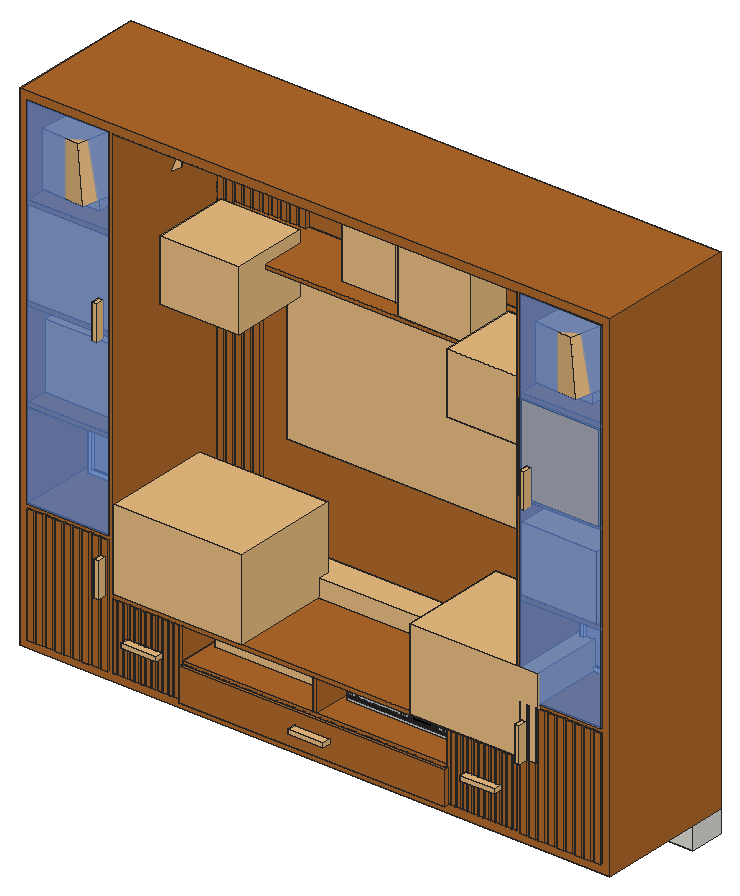
# SketchUp Ruby script. Lengths in millimetres.
U = 1.mm
M = Sketchup.active_model
def pt(a) = Geom::Point3d.new(a.map { |v| v * U })
def face(e, loops, mat)
  f = e.add_face(loops[0].map { |a| pt(a) })
  loops[1..].each { |l| e.add_face(l.map { |a| pt(a) }).erase! }
  f.material = f.back_material = mat if mat
  f
end
# faces: each face lists its corners as indices into pts; further lists are holes
def faces(e, pts, list, mat = nil) = list.each { |f| face(e, (f[0].is_a?(Array) ? f : [f]).map { |l| l.map { |i| pts[i] } }, mat) }
# xy, xz, yz: faces in a plane at the given z, y or x. An outline is a flat list of corners, or four numbers for a rectangle; further outlines are holes
def ring(l) = l.size == 4 ? [[l[0], l[1]], [l[2], l[1]], [l[2], l[3]], [l[0], l[3]]] : l.each_slice(2).to_a
def flat(e, list, mat, &to3) = list.each { |f| face(e, (f[0].is_a?(Array) ? f : [f]).map { |l| ring(l).map { |u, v| to3.(u, v) } }, mat) }
def xy(e, z, list, mat = nil) = flat(e, list, mat) { |x, y| [x, y, z] }
def xz(e, y, list, mat = nil) = flat(e, list, mat) { |x, z| [x, y, z] }
def yz(e, x, list, mat = nil) = flat(e, list, mat) { |y, z| [x, y, z] }
def lines(e, pts, list) = list.each { |a, b| e.add_line(pt(pts[a]), pt(pts[b])) }
# prism: a flat outline (further loops are holes) pulled along v
def prism(e, loops, v, mat = nil)
  f = face(e, loops, mat); d = Geom::Vector3d.new(v.map { |x| x * U })
  f.pushpull(f.normal.samedirection?(d) ? d.length : -d.length)
end
def box(e, o, s, mat = nil) = prism(e, [[o, [o[0] + s[0], o[1], o[2]], [o[0] + s[0], o[1] + s[1], o[2]], [o[0], o[1] + s[1], o[2]]]], [0, 0, s[2]], mat)
def at(x, y, z, deg = 0) = Geom::Transformation.translation(pt([x, y, z])) * Geom::Transformation.rotation(ORIGIN, Z_AXIS, deg.degrees)
def axes(o, x, y, z) = Geom::Transformation.new([*x, 0, *y, 0, *z, 0, *pt(o).to_a, 1])
def part(name) = M.definitions.add(name)
# library, detail: a bought-in or finely detailed component or shape, given as its bounding box
def library(name, o, s) = part(name).tap { |d| box(d.entities, o, s) }
def detail(e, o, s) = box(e.add_group.entities, o, s)
def put(e, d, t, mat = nil) = e.add_instance(d, t).tap { |i| i.material = mat if mat }
def group(e, t, mat = nil) = e.add_group.tap { |g| g.transformation = t; g.material = mat if mat }.entities
root = M.entities
M.materials.add("Material__1").color = [190, 136, 85]
M.materials.add("Material__2").color = [51, 42, 44]
M.materials.add("Material__3").color = [119, 136, 107]
M.materials.add("Paintiing ").color = [206, 175, 155]
M.materials.add("[0131_Silver]").color = [192, 192, 192]
M.materials.add("[0136_Charcoal]").color = [35, 35, 35]
M.materials.add("[0137_Black]").color = [0, 0, 0]
M.materials.add("[Marble Carrara Gold Floor Tile]").color = [225, 223, 217]
M.materials.add("[Translucent Glass Blue]").color = [100, 149, 237]
M.materials["[Translucent Glass Blue]"].alpha = 0.5
M.materials.add("[Wood Bamboo]").color = [177, 105, 43]
c1 = part("Circular disc")
prism(c1.entities,[[[0,76.2,-25],[2.6,95.9,-25],[10.2,114.3,-25],[22.3,130.1,-25],[38.1,142.2,-25],[56.5,149.8,-25],[76.2,152.4,-25],[95.9,149.8,-25],[114.3,142.2,-25],[130.1,130.1,-25],[142.2,114.3,-25],[149.8,95.9,-25],[152.4,76.2,-25],[149.8,56.5,-25],[142.2,38.1,-25],[130.1,22.3,-25],[114.3,10.2,-25],[95.9,2.6,-25],[76.2,0,-25],[56.5,2.6,-25],[38.1,10.2,-25],[22.3,22.3,-25],[10.2,38.1,-25],[2.6,56.5,-25]]],[0,0,13])
c2 = library("1-POIGNEE CLC2\#1",[-77,-9.5,0],[154,19,36])
c3 = library("1-POIGNEE CLC2\#2",[-77,-9.5,0],[154,19,36])
c4 = library("1-POIGNEE CLC2\#3",[-77,-9.5,0],[154,19,36])
c5 = library("download?mid=50c7180b9fccec56d493bfe20f94b6ab&ctyp=sp&cv=p8.",[3795.5,1113.3,453.6],[1898.6,14.5,1067.8])
c6 = library("cay+chuoi",[682.9,499.4,13.3],[1066,1159.4,897.8])
c7 = library("\#2",[-3043.7,-3043.7,2890.5],[6087.4,6087.4,441.9])
c8 = library("\#4",[-4912.8,-5236.5,-6012.5],[10484.7,6383.2,12002.4])
c9 = part("\#3")
put(c9.entities,c8,axes([-9.5,7866.8,0],[1.36765,0,0],[0,1.36765,0],[0,0,1.36765]),"Material__3")
c10 = library("\#1",[-4421.5,-4421.5,0],[8843,8843,3556])
c11 = part("9")
put(c11.entities,c7,at(-506.5,-626.4,0),"Material__2")
put(c11.entities,c9,axes([448.8,-828,1023.3],[0.29694,0.9549,0],[-0.21403,0.06656,0.97456],[0.9306,-0.28939,0.22414]))
put(c11.entities,c10,at(-506.5,-626.4,0),"Material__1")
c12 = library("Hanging potted plant",[2125.6,-54.2,204.6],[849,690.2,1168.3])
c13 = library("Plant (3)",[-393.8,66.9,0],[2990,2448.2,4692.7])
c14 = library("Pot Wired",[-4344.5,-4889.6,-19],[9129.4,9129.4,7192.3])
c15 = library("Seated statue",[0,0,0],[467.3,421.3,661.2])
c16 = part("Framed panel")
xy(c16.entities,0,[[[0,0,1153.7,1374.2],[66.8,66.8,1086.8,1307.4]]])
xy(c16.entities,0,[[66.8,66.8,1086.8,1307.4]],"Paintiing ")
xy(c16.entities,10,[[[0,0,1153.7,1374.2],[66.8,66.8,1086.8,1307.4]]])
xz(c16.entities,0,[[0,0,1153.7,10]])
xz(c16.entities,66.8,[[66.8,0,1086.8,10]])
xz(c16.entities,1307.4,[[66.8,0,1086.8,10]])
xz(c16.entities,1374.2,[[0,0,1153.7,10]])
yz(c16.entities,0,[[0,0,1374.2,10]])
yz(c16.entities,66.8,[[66.8,0,1307.4,10]])
yz(c16.entities,1086.8,[[66.8,0,1307.4,10]])
yz(c16.entities,1153.7,[[0,0,1374.2,10]])
c17 = library("SetUp-Box",[-7.9,-1.3,-4],[171.7,230.9,39.1])
c18 = library("Ganesha+-+An+Do+Giao",[214.1,-280.3,-3.5],[241.1,146.8,312])
c19 = library("Samsung+soundbar",[-449.8,4.4,0],[1488,131,78.2])
c20 = part("Untitled")
xy(c20.entities,695.4,[[-2447.8,-1052.2,-473,-61.6]],"[0131_Silver]")
xy(c20.entities,720.8,[[-2447.8,-1058.5,-473,-1052.2]],"[0136_Charcoal]")
xy(c20.entities,740.9,[[-1374.3,-1058.5,-1037.8,-1052.2]],"[0136_Charcoal]")
xy(c20.entities,758.1,[[-913.8,-1077.6,-831.3,-1058.5]],"[0131_Silver]")
xy(c20.entities,758.3,[[-636.9,-1077.6,-579.8,-1058.5]],"[0131_Silver]")
xy(c20.entities,762.4,[[-1518.7,-1077.6,-1436.1,-1058.5]],"[0131_Silver]")
xy(c20.entities,762.6,[[-714.1,-1077.6,-663.3,-1058.5]],"[0131_Silver]")
xy(c20.entities,762.9,[[-2398.3,-1077.6,-2315.7,-1058.5]],"[0131_Silver]")
xy(c20.entities,765.2,[[-807.4,-1077.6,-743.9,-1058.5]],"[0131_Silver]")
xy(c20.entities,768.4,[[-707.6,-1077.6,-669.5,-1064.9]],"[0131_Silver]")
xy(c20.entities,774.7,[[-707.6,-1077.6,-669.5,-1064.9]],"[0131_Silver]")
xy(c20.entities,781.5,[[-1518.7,-1077.6,-1436.1,-1058.5]],"[0131_Silver]")
xy(c20.entities,781.6,[[-714.1,-1077.6,-663.3,-1058.5]],"[0131_Silver]")
xy(c20.entities,781.9,[[-2398.3,-1077.6,-2315.7,-1058.5]],"[0131_Silver]")
xy(c20.entities,783.5,[[-913.8,-1077.6,-831.3,-1058.5]],"[0131_Silver]")
xy(c20.entities,783.7,[[-636.9,-1077.6,-634,-1058.5],[-634,-1077.6,-631.2,-1058.5],[-631.2,-1077.6,-586.7,-1058.5],[-586.7,-1077.6,-583.2,-1058.5],[-583.2,-1077.6,-579.8,-1058.5]],"[0131_Silver]")
xy(c20.entities,784.3,[[-807.4,-1077.6,-743.9,-1058.5]],"[0131_Silver]")
xy(c20.entities,791.7,[[-1374.3,-1058.5,-1037.8,-1052.2]],"[0136_Charcoal]")
xy(c20.entities,835.2,[[-2425.6,-1058.5,-488.8,-1052.2]],"[0136_Charcoal]")
xy(c20.entities,853.4,[[-2426.6,-1052.2,-502.6,-61.6]],"[0131_Silver]")
xz(c20.entities,-1077.6,[[-913.8,758.1,-831.3,783.5],[-636.9,758.3,-636.9,783.7,-634,783.7,-634,764.7,-583.2,764.7,-583.2,783.7,-579.8,783.7,-579.8,758.3],[-1518.7,762.4,-1436.1,781.5],[[-714.1,762.6,-663.3,781.6],[-707.6,768.4,-669.5,774.7]],[-2398.3,762.9,-2315.7,781.9],
  [-807.4,765.2,-743.9,784.3],[-631.2,777.4,-586.7,783.7]],"[0131_Silver]")
xz(c20.entities,-1058.5,[[-2259.9,752,-1548.7,790.1]],"[0131_Silver]")
xz(c20.entities,-1058.5,[[[-2447.8,720.8,-2447.8,816,-2447.6,818.8,-2447,821.5,-2446,824.1,-2444.7,826.5,-2443,828.7,-2441.1,830.7,-2438.9,832.4,-2436.4,833.7,-2433.8,834.7,-2431.1,835.2,-2428.3,835.4,-2425.6,835.2,-488.8,835.2,-486.5,835.1,-484.1,834.5,-481.9,833.7,-479.9,832.5,-478,831.1,-476.4,829.4,-475,827.4,-473.9,825.3,-473.2,823.1,-472.7,820.7,-472.7,818.4,-473,816,-473,720.8],[-2259.9,752,-1548.7,790.1],[-1374.3,740.9,-1037.8,791.7],[-913.8,758.1,-831.3,783.5],[-2398.3,762.9,-2315.7,781.9],[-1518.7,762.4,-1436.1,781.5],[-636.9,758.3,-579.8,783.7],[-807.4,765.2,-743.9,784.3],[-714.1,762.6,-663.3,781.6]]],"[0136_Charcoal]")
xz(c20.entities,-1052.2,[[-2447.8,695.4,-473,720.8],[-2436.4,833.7,-2433.8,834.7,-2431.1,835.2,-2428.3,835.4,-2425.6,835.2,-488.8,835.2,-486.5,835.1,-484.1,834.5,-484.1,847.2,-485.5,848.2,-486.9,849.1,-488.3,849.9,-489.8,850.6,-491.3,851.2,-492.9,851.8,-494.5,852.3,-496.1,852.7,-497.7,853,-499.3,853.2,-500.9,853.3,-502.6,853.4,-2426.6,853.4,-2428.2,853.2,-2429.8,852.9,-2431.3,852.3,-2432.6,851.4,-2433.9,850.4,-2434.9,849.2,-2435.7,847.8,-2436.4,846.3,-2436.8,844.8,-2436.9,843.2,-2436.8,841.6,-2436.4,840]],"[0131_Silver]")
xz(c20.entities,-1052.2,[[-1374.3,740.9,-1037.8,791.7]],"[0137_Black]")
xz(c20.entities,-61.6,[[-2447.8,695.4,-2447.8,816,-2447.6,818.8,-2447,821.5,-2446,824.1,-2444.7,826.5,-2443,828.7,-2441.1,830.7,-2438.9,832.4,-2436.4,833.7,-2433.8,834.7,-2431.1,835.2,-2428.3,835.4,-2425.6,835.2,-488.8,835.2,-486.5,835.1,-484.1,834.5,-481.9,833.7,-479.9,832.5,-478,831.1,-476.4,829.4,-475,827.4,-473.9,825.3,-473.2,823.1,-472.7,820.7,-472.7,818.4,-473,816,-473,695.4],[-2436.4,833.7,-2436.4,840,-2436.8,841.6,-2436.9,843.2,-2436.8,844.8,-2436.4,846.3,-2435.7,847.8,-2434.9,849.2,-2433.9,850.4,-2432.6,851.4,-2431.3,852.3,-2429.8,852.9,-2428.2,853.2,-2426.6,853.4,-502.6,853.4,-500.9,853.3,-499.3,853.2,-497.7,853,-496.1,852.7,-494.5,852.3,-492.9,851.8,-491.3,851.2,-489.8,850.6,-488.3,849.9,-486.9,849.1,-485.5,848.2,-484.1,847.2,-484.1,834.5,-486.5,835.1,-488.8,835.2,-2425.6,835.2,-2428.3,835.4,-2431.1,835.2,-2433.8,834.7]],"[0131_Silver]")
yz(c20.entities,-2447.8,[[-1052.2,695.4,-61.6,727.1],[-1058.5,720.8,-1052.2,720.8,-1052.2,727.1,-61.6,727.1,-61.6,816,-1058.5,816]],"[0131_Silver]")
yz(c20.entities,-2436.4,[[-1052.2,833.7,-61.6,840]],"[0131_Silver]")
yz(c20.entities,-2398.3,[[-1077.6,762.9,-1058.5,781.9]],"[0131_Silver]")
yz(c20.entities,-2315.7,[[-1077.6,762.9,-1058.5,781.9]],"[0131_Silver]")
yz(c20.entities,-1518.7,[[-1077.6,762.4,-1058.5,781.5]],"[0131_Silver]")
yz(c20.entities,-1436.1,[[-1077.6,762.4,-1058.5,781.5]],"[0131_Silver]")
yz(c20.entities,-1374.3,[[-1058.5,740.9,-1052.2,791.7]],"[0136_Charcoal]")
yz(c20.entities,-1037.8,[[-1058.5,740.9,-1052.2,791.7]],"[0136_Charcoal]")
yz(c20.entities,-913.8,[[-1077.6,758.1,-1058.5,783.5]],"[0131_Silver]")
yz(c20.entities,-831.3,[[-1077.6,758.1,-1058.5,783.5]],"[0131_Silver]")
yz(c20.entities,-807.4,[[-1077.6,765.2,-1058.5,784.3]],"[0131_Silver]")
yz(c20.entities,-743.9,[[-1077.6,765.2,-1058.5,784.3]],"[0131_Silver]")
yz(c20.entities,-714.1,[[-1077.6,762.6,-1058.5,781.6]],"[0131_Silver]")
yz(c20.entities,-707.6,[[-1077.6,768.4,-1064.9,774.7]],"[0131_Silver]")
yz(c20.entities,-669.5,[[-1077.6,768.4,-1064.9,774.7]],"[0131_Silver]")
yz(c20.entities,-663.3,[[-1077.6,762.6,-1058.5,781.6]],"[0131_Silver]")
yz(c20.entities,-636.9,[[-1077.6,758.3,-1058.5,783.7]],"[0131_Silver]")
yz(c20.entities,-579.8,[[-1077.6,758.3,-1058.5,783.7]],"[0131_Silver]")
yz(c20.entities,-484.1,[[-1052.2,834.5,-61.6,847.2]],"[0131_Silver]")
yz(c20.entities,-473,[[-1052.2,695.4,-61.6,727.1],[-1058.5,720.8,-1058.5,816,-61.6,816,-61.6,727.1,-1052.2,727.1,-1052.2,720.8]],"[0131_Silver]")
yz(c20.entities,-472.7,[[-1058.5,818.4,-61.6,820.7]],"[0131_Silver]")
p = [[-2447.8,-1058.5,816],[-2447.8,-61.6,816],[-2447.6,-61.6,818.8],[-2447.6,-1058.5,818.8],[-472.7,-1058.5,818.4],[-472.7,-61.6,818.4],
  [-473,-61.6,816],[-473,-1058.5,816],[-2447,-61.6,821.5],[-2447,-1058.5,821.5],[-473.2,-1058.5,823.1],[-473.2,-61.6,823.1],
  [-472.7,-61.6,820.7],[-472.7,-1058.5,820.7],[-2446,-61.6,824.1],[-2446,-1058.5,824.1],[-473.9,-1058.5,825.3],[-473.9,-61.6,825.3],
  [-2444.7,-61.6,826.5],[-2444.7,-1058.5,826.5],[-475,-1058.5,827.4],[-475,-61.6,827.4],[-2443,-61.6,828.7],[-2443,-1058.5,828.7],
  [-476.4,-1058.5,829.4],[-476.4,-61.6,829.4],[-2441.1,-61.6,830.7],[-2441.1,-1058.5,830.7],[-478,-1058.5,831.1],[-478,-61.6,831.1],
  [-2438.9,-61.6,832.4],[-2438.9,-1058.5,832.4],[-479.9,-1058.5,832.5],[-479.9,-61.6,832.5],[-2436.4,-61.6,833.7],[-2436.4,-1052.2,833.7],
  [-2436.4,-1058.5,833.7],[-481.9,-1058.5,833.7],[-481.9,-61.6,833.7],[-2433.8,-1052.2,834.7],[-2433.8,-1058.5,834.7],[-484.1,-1052.2,834.5],
  [-484.1,-61.6,834.5],[-484.1,-1058.5,834.5],[-486.5,-1052.2,835.1],[-486.5,-1058.5,835.1],[-2431.1,-1052.2,835.2],[-2431.1,-1058.5,835.2],
  [-488.8,-1052.2,835.2],[-488.8,-1058.5,835.2],[-2428.3,-1052.2,835.4],[-2428.3,-1058.5,835.4],[-2425.6,-1052.2,835.2],[-2425.6,-1058.5,835.2],
  [-2436.8,-61.6,841.6],[-2436.4,-61.6,840],[-2436.4,-1052.2,840],[-2436.8,-1052.2,841.6],[-2436.9,-61.6,843.2],[-2436.9,-1052.2,843.2],
  [-2436.8,-61.6,844.8],[-2436.8,-1052.2,844.8],[-2436.4,-61.6,846.3],[-2436.4,-1052.2,846.3],[-2435.7,-61.6,847.8],[-2435.7,-1052.2,847.8],
  [-484.1,-61.6,847.2],[-485.5,-61.6,848.2],[-485.5,-1052.2,848.2],[-484.1,-1052.2,847.2],[-2434.9,-61.6,849.2],[-2434.9,-1052.2,849.2],
  [-486.9,-61.6,849.1],[-486.9,-1052.2,849.1],[-488.3,-61.6,849.9],[-488.3,-1052.2,849.9],[-2433.9,-61.6,850.4],[-2433.9,-1052.2,850.4],
  [-489.8,-61.6,850.6],[-489.8,-1052.2,850.6],[-2432.6,-61.6,851.4],[-2432.6,-1052.2,851.4],[-491.3,-61.6,851.2],[-491.3,-1052.2,851.2],
  [-492.9,-61.6,851.8],[-492.9,-1052.2,851.8],[-2431.3,-61.6,852.3],[-2431.3,-1052.2,852.3],[-494.5,-61.6,852.3],[-494.5,-1052.2,852.3],
  [-2429.8,-61.6,852.9],[-2429.8,-1052.2,852.9],[-496.1,-61.6,852.7],[-496.1,-1052.2,852.7],[-497.7,-61.6,853],[-497.7,-1052.2,853],
  [-2428.2,-61.6,853.2],[-2428.2,-1052.2,853.2],[-499.3,-61.6,853.2],[-499.3,-1052.2,853.2],[-2426.6,-61.6,853.4],[-2426.6,-1052.2,853.4],
  [-500.9,-61.6,853.3],[-500.9,-1052.2,853.3],[-502.6,-61.6,853.4],[-502.6,-1052.2,853.4],[-486.5,-620.4,835.1],[-488.8,-620.4,835.2],
  [-2425.6,-620.4,835.2],[-2428.3,-620.4,835.4],[-2431.1,-620.4,835.2],[-2433.8,-620.4,834.7]]
faces(c20.entities,p,[[0,1,2,3],[4,5,6,7],[3,2,8,9],[10,11,12,13],[9,8,14,15],[16,17,11,10],[15,14,18,19],[20,21,17,16],
  [19,18,22,23],[24,25,21,20],[23,22,26,27],[28,29,25,24],[27,26,30,31],[32,33,29,28],[31,30,34,35,36],[37,38,33,32],
  [41,42,38,37,43],[54,55,56,57],[58,54,57,59],[60,58,59,61],[62,60,61,63],[64,62,63,65],[66,67,68,69],[70,64,65,71],
  [67,72,73,68],[72,74,75,73],[76,70,71,77],[74,78,79,75],[80,76,77,81],[78,82,83,79],[82,84,85,83],[86,80,81,87],
  [84,88,89,85],[90,86,87,91],[88,92,93,89],[92,94,95,93],[96,90,91,97],[94,98,99,95],[100,96,97,101],[98,102,103,99],
  [102,104,105,103]],"[0131_Silver]")
faces(c20.entities,p,[[39,35,36,40],[41,44,45,43],[46,39,40,47],[44,48,49,45],[50,46,47,51],[52,50,51,53]])
lines(c20.entities,p,[[106,44],[107,48],[108,52],[109,50],[110,46],[111,39]])
c21 = library("1-POIGNEE CLC2\#4",[-77,-9.5,0],[154,19,36])
c22 = part("louvers")
box(c22.entities,[0,-2,0],[18.7,2,291])
box(c22.entities,[24.8,-2,0],[18.7,2,291])
box(c22.entities,[49.5,-2,0],[18.7,2,291])
box(c22.entities,[74.3,-2,0],[18.7,2,291])
box(c22.entities,[99,-2,0],[18.7,2,291])
box(c22.entities,[123.8,-2,0],[18.7,2,291])
box(c22.entities,[148.5,-2,0],[18.7,2,291])
box(c22.entities,[173.3,-2,0],[18.7,2,291])
box(c22.entities,[198,-2,0],[18.7,2,291])
box(c22.entities,[222.8,-2,0],[18.7,2,291])
box(c22.entities,[247.5,-2,0],[18.7,2,291])
box(c22.entities,[272.3,-2,0],[18.7,2,291])
c23 = part("Group\#24")
xz(c23.entities,0,[[18.7,0,291,291]])
put(c23.entities,c22,at(0,0,0))
c24 = part("Group\#48")
box(c24.entities,[0,-18,0],[29.8,18,490.1],"[Wood Bamboo]")
c25 = part("Group\#36")
box(c25.entities,[0,-18,0],[29.8,18,490.1],"[Wood Bamboo]")
xy(root,36,[[1882,18,1900,609.6]])
xy(root,327,[[1882,18,1900,609.6]])
xz(root,18,[[1882,36,1900,327]],"[Wood Bamboo]")
xz(root,609.6,[[1882,36,1900,327]])
yz(root,1882,[[18,36,609.6,327]],"[Wood Bamboo]")
yz(root,1900,[[18,36,609.6,327]],"[Wood Bamboo]")
put(root,c1,at(137.3,237.6,2164))
put(root,c1,at(680.6,237.6,2164))
put(root,c1,at(1223.8,237.6,2164))
put(root,c1,at(1767,237.6,2164))
put(root,c1,at(2310.3,237.6,2164))
put(root,c2,axes([551.5,16,181.5],[1,0,0],[0,0,1],[0,-1,0]))
put(root,c2,axes([2042.5,18,181.5],[1,0,0],[0,0,1],[0,-1,0]))
put(root,c3,axes([1301.1,0,112.4],[1,0,0],[0,0,1],[0,-1,0]))
put(root,c4,axes([2225.6,11,409.7],[0,0,1],[-1,0,0],[0,-1,0]))
put(root,c4,axes([369.9,11,409.7],[0,0,1],[-1,0,0],[0,-1,0]))
put(root,c5,axes([-1630.5,-506,524.1],[0.61563,0,0],[0,1,0],[0,0,0.62]))
put(root,c6,axes([45.1,-186.8,339.7],[0.5328,0,0],[0,0.41,0],[0,0,0.3953]))
put(root,c11,axes([207.3,253.2,1782.1],[0.02083,0,0],[0,0.03139,0],[0,0,0.02649]))
put(root,c11,axes([2380.3,253.2,1782.1],[0.02083,0,0],[0,0.03139,0],[0,0,0.02649]))
put(root,c12,axes([-375.3,194.2,1409.7],[0.41,0,0],[0,0.48917,0],[0,0,0.22897]))
put(root,c12,axes([891.4,194.2,1409.7],[0.41,0,0],[0,0.48917,0],[0,0,0.22897]))
put(root,c13,axes([1475,304.4,1673.9],[0.10781,0,0],[0,0.07727,0],[0,0,0.08155]))
put(root,c14,axes([204.9,247.9,973.8],[0.03889,0,0],[0,0.02878,0],[0,0,0.04037]))
put(root,c14,axes([2358.2,159,973.8],[0.03889,0,0],[0,0.02878,0],[0,0,0.04037]))
put(root,c15,axes([36,18,1373],[0.75963,0,0],[0,1,0],[0,0,0.57776]))
put(root,c15,axes([2198.1,14.7,1366.3],[0.75963,0,0],[0,1,0],[0,0,0.57776]))
put(root,c16,axes([373,323.8,573],[-0.26862,0,0],[0,0,0.24752],[0,-1,0]))
put(root,c16,axes([2541.4,323.8,573],[-0.26862,0,0],[0,0,0.24752],[0,-1,0]))
put(root,c17,axes([763.6,165.5,189.6],[3,0,0],[0,1,0],[0,0,2]))
put(root,c18,at(910.9,663.6,1673.9))
put(root,c6,axes([1358.3,-193.8,332.8],[0.5328,0,0],[0,0.41,0],[0,0,0.3953]))
put(root,c19,axes([1059.8,437.3,345],[0.7387,0,0],[0,1,0],[0,0,1]))
put(root,c20,axes([1982.8,552.6,-129.4],[0.2666,0,0],[0,0.3775,0],[0,0,0.46]))
put(root,c21,axes([360.4,12,1419.8],[0,0,1],[-1,0,0],[0,-1,0]))
put(root,c21,axes([2246.4,12,1419.8],[0,0,1],[-1,0,0],[0,-1,0]))
g1 = group(root,at(700,18,36),"[Wood Bamboo]")
box(g1,[0,0,0],[18,591.6,291])
put(root,c23,at(409,18,36),"[Wood Bamboo]")
g2 = group(root,at(1291,18,181.5),"[Wood Bamboo]")
xy(g2,145.5,[[0,0,18,591.6]])
g3 = group(g2,at(0,0,0))
xy(g3,9,[[0,0,18,591.6]])
xz(g3,0,[[0,9,18,145.5]])
xz(g3,591.6,[[0,9,18,145.5]])
yz(g3,0,[[0,9,591.6,145.5]])
yz(g3,18,[[0,9,591.6,145.5]])
g4 = group(root,at(1463.5,18,181.5),"[Wood Bamboo]")
box(g4,[-745.5,0,-9],[1164,591.6,18])
g5 = group(root,at(0,627.6,-100),"[Marble Carrara Gold Floor Tile]")
box(g5,[0,-150,0],[2600,150,100])
g6 = group(root,at(36,18,573),"[Translucent Glass Blue]")
box(g6,[-3,-6,-3],[361,6,1597])
g7 = group(root,at(2209,18,573),"[Translucent Glass Blue]")
box(g7,[-3,-6,-3],[361,6,1597])
g8 = group(root,at(0,627.6,0),"[Wood Bamboo]")
xy(g8,0,[[0,-609.6,2600,0]],"[Wood Bamboo]")
xy(g8,36,[[409,-609.6,2191,-18]],"[Wood Bamboo]")
xy(g8,327,[[409,-609.6,2191,-18]],"[Wood Bamboo]")
xy(g8,345,[[409,-609.6,2191,-18]],"[Wood Bamboo]")
xy(g8,573,[[36,-609.6,391,-18],[2209,-609.6,2564,-18]],"[Wood Bamboo]")
xy(g8,955,[[36,-609.6,391,-18],[2209,-609.6,2564,-18]],"[Wood Bamboo]")
xy(g8,973,[[36,-609.6,391,-18],[2209,-609.6,2564,-18]],"[Wood Bamboo]")
xy(g8,1355,[[36,-609.6,391,-18],[2209,-609.6,2564,-18]],"[Wood Bamboo]")
xy(g8,1373,[[36,-609.6,391,-18],[2209,-609.6,2564,-18]],"[Wood Bamboo]")
xy(g8,1755,[[36,-609.6,391,-18],[2209,-609.6,2564,-18]],"[Wood Bamboo]")
xy(g8,1773,[[36,-609.6,391,-18],[2209,-609.6,2564,-18]],"[Wood Bamboo]")
xy(g8,2164,[[36,-609.6,391,-18],[409,-609.6,409,-18,769,-18,769,-36,798.8,-36,798.8,-18,2191,-18,2191,-609.6],[2209,-609.6,2564,-18],[769,-36,798.8,-18]],"[Wood Bamboo]")
xy(g8,2200,[[0,-609.6,2600,0]],"[Wood Bamboo]")
xz(g8,-609.6,[[[0,0,2600,2200],[409,36,2191,2164],[2209,1773,2564,2164],[36,1773,391,2164],[2209,1373,2564,1755],[2209,973,2564,1355],[2209,573,2564,955],[36,1373,391,1755],[36,573,391,955],[36,973,391,1355]],[409,327,2191,345]],"[Wood Bamboo]")
xz(g8,-18,[[798.8,1673.9,799.3,2164]])
xz(g8,-18,[[409,36,2191,327],[36,573,391,955],[2209,573,2564,955],[36,973,391,1355],[2209,973,2564,1355],
  [36,1373,391,1755],[2209,1373,2564,1755],[36,1773,391,2164],[2209,1773,2564,2164]],"[Wood Bamboo]")
xz(g8,0,[[0,0,2600,2200]],"[Wood Bamboo]")
yz(g8,0,[[-609.6,0,0,2200]],"[Wood Bamboo]")
yz(g8,36,[[-609.6,573,-18,955],[-609.6,973,-18,1355],[-609.6,1373,-18,1755],[-609.6,1773,-18,2164]],"[Wood Bamboo]")
yz(g8,391,[[-609.6,573,-18,955],[-609.6,973,-18,1355],[-609.6,1373,-18,1755],[-609.6,1773,-18,2164]],"[Wood Bamboo]")
yz(g8,409,[[-609.6,36,-18,327],[-609.6,345,-18,2164]],"[Wood Bamboo]")
yz(g8,2191,[[-609.6,36,-18,327],[-609.6,345,-18,2164]],"[Wood Bamboo]")
yz(g8,2209,[[-609.6,573,-18,955],[-609.6,973,-18,1355],[-609.6,1373,-18,1755],[-609.6,1773,-18,2164]],"[Wood Bamboo]")
yz(g8,2564,[[-609.6,573,-18,955],[-609.6,973,-18,1355],[-609.6,1373,-18,1755],[-609.6,1773,-18,2164]],"[Wood Bamboo]")
yz(g8,2600,[[-609.6,0,0,2200]],"[Wood Bamboo]")
p = [[438.8,-18,2164],[438.8,-18,345]]
lines(g8,p,[[0,1]])
g9 = group(g8,at(36,-609.6,36))
xz(g9,0,[[30.6,0,355,519]])
g10 = group(g9,at(0,0,0))
xy(g10,0,[[0,-7,30.6,0]])
xy(g10,519,[[0,-7,30.6,0]])
xz(g10,-7,[[0,0,30.6,519]])
xz(g10,0,[[0,0,30.6,519]])
yz(g10,0,[[-7,0,0,519]],"[Wood Bamboo]")
yz(g10,30.6,[[-7,0,0,519]],"[Wood Bamboo]")
g11 = group(g9,at(40.5,0,0))
xy(g11,0,[[0,-7,30.6,0]])
xy(g11,519,[[0,-7,30.6,0]])
xz(g11,-7,[[0,0,30.6,519]])
xz(g11,0,[[0,0,30.6,519]])
yz(g11,0,[[-7,0,0,519]],"[Wood Bamboo]")
yz(g11,30.6,[[-7,0,0,519]],"[Wood Bamboo]")
g12 = group(g9,at(81.1,0,0))
xy(g12,0,[[0,-7,30.6,0]])
xy(g12,519,[[0,-7,30.6,0]])
xz(g12,-7,[[0,0,30.6,519]])
xz(g12,0,[[0,0,30.6,519]])
yz(g12,0,[[-7,0,0,519]],"[Wood Bamboo]")
yz(g12,30.6,[[-7,0,0,519]],"[Wood Bamboo]")
g13 = group(g9,at(121.6,0,0))
xy(g13,0,[[0,-7,30.6,0]])
xy(g13,519,[[0,-7,30.6,0]])
xz(g13,-7,[[0,0,30.6,519]])
xz(g13,0,[[0,0,30.6,519]])
yz(g13,0,[[-7,0,0,519]],"[Wood Bamboo]")
yz(g13,30.6,[[-7,0,0,519]],"[Wood Bamboo]")
g14 = group(g9,at(162.2,0,0))
xy(g14,0,[[0,-7,30.6,0]])
xy(g14,519,[[0,-7,30.6,0]])
xz(g14,-7,[[0,0,30.6,519]])
xz(g14,0,[[0,0,30.6,519]])
yz(g14,0,[[-7,0,0,519]],"[Wood Bamboo]")
yz(g14,30.6,[[-7,0,0,519]],"[Wood Bamboo]")
g15 = group(g9,at(202.7,0,0))
xy(g15,0,[[0,-7,30.6,0]])
xy(g15,519,[[0,-7,30.6,0]])
xz(g15,-7,[[0,0,30.6,519]])
xz(g15,0,[[0,0,30.6,519]])
yz(g15,0,[[-7,0,0,519]],"[Wood Bamboo]")
yz(g15,30.6,[[-7,0,0,519]],"[Wood Bamboo]")
g16 = group(g9,at(243.3,0,0))
xy(g16,0,[[0,-7,30.6,0]])
xy(g16,519,[[0,-7,30.6,0]])
xz(g16,-7,[[0,0,30.6,519]])
xz(g16,0,[[0,0,30.6,519]])
yz(g16,0,[[-7,0,0,519]],"[Wood Bamboo]")
yz(g16,30.6,[[-7,0,0,519]],"[Wood Bamboo]")
g17 = group(g9,at(283.8,0,0))
xy(g17,0,[[0,-7,30.6,0]])
xy(g17,519,[[0,-7,30.6,0]])
xz(g17,-7,[[0,0,30.6,519]])
xz(g17,0,[[0,0,30.6,519]])
yz(g17,0,[[-7,0,0,519]],"[Wood Bamboo]")
yz(g17,30.6,[[-7,0,0,519]],"[Wood Bamboo]")
g18 = group(g9,at(324.4,0,0))
xy(g18,0,[[0,-7,30.6,0]])
xy(g18,519,[[0,-7,30.6,0]])
xz(g18,-7,[[0,0,30.6,519]])
xz(g18,0,[[0,0,30.6,519]])
yz(g18,0,[[-7,0,0,519]],"[Wood Bamboo]")
yz(g18,30.6,[[-7,0,0,519]],"[Wood Bamboo]")
g19 = group(g8,at(2209,-609.6,36))
xz(g19,0,[[0,0,355,519]])
g20 = group(g8,at(2209,-609.6,36))
p = [[355,0,0],[355,0,519],[30.6,0,519],[30.6,0,0]]
lines(g20,p,[[0,1],[1,2],[2,3],[3,0]])
g21 = group(g20,at(0,0,0))
xy(g21,0,[[0,-7,30.6,0]])
xy(g21,519,[[0,-7,30.6,0]])
xz(g21,-7,[[0,0,30.6,519]])
xz(g21,0,[[0,0,30.6,519]])
yz(g21,0,[[-7,0,0,519]],"[Wood Bamboo]")
yz(g21,30.6,[[-7,0,0,519]],"[Wood Bamboo]")
g22 = group(g20,at(40.5,0,0))
xy(g22,0,[[0,-7,30.6,0]])
xy(g22,519,[[0,-7,30.6,0]])
xz(g22,-7,[[0,0,30.6,519]])
xz(g22,0,[[0,0,30.6,519]])
yz(g22,0,[[-7,0,0,519]],"[Wood Bamboo]")
yz(g22,30.6,[[-7,0,0,519]],"[Wood Bamboo]")
g23 = group(g20,at(81.1,0,0))
xy(g23,0,[[0,-7,30.6,0]])
xy(g23,519,[[0,-7,30.6,0]])
xz(g23,-7,[[0,0,30.6,519]])
xz(g23,0,[[0,0,30.6,519]])
yz(g23,0,[[-7,0,0,519]],"[Wood Bamboo]")
yz(g23,30.6,[[-7,0,0,519]],"[Wood Bamboo]")
g24 = group(g20,at(121.6,0,0))
xy(g24,0,[[0,-7,30.6,0]])
xy(g24,519,[[0,-7,30.6,0]])
xz(g24,-7,[[0,0,30.6,519]])
xz(g24,0,[[0,0,30.6,519]])
yz(g24,0,[[-7,0,0,519]],"[Wood Bamboo]")
yz(g24,30.6,[[-7,0,0,519]],"[Wood Bamboo]")
g25 = group(g20,at(162.2,0,0))
xy(g25,0,[[0,-7,30.6,0]])
xy(g25,519,[[0,-7,30.6,0]])
xz(g25,-7,[[0,0,30.6,519]])
xz(g25,0,[[0,0,30.6,519]])
yz(g25,0,[[-7,0,0,519]],"[Wood Bamboo]")
yz(g25,30.6,[[-7,0,0,519]],"[Wood Bamboo]")
g26 = group(g20,at(202.7,0,0))
xy(g26,0,[[0,-7,30.6,0]])
xy(g26,519,[[0,-7,30.6,0]])
xz(g26,-7,[[0,0,30.6,519]])
xz(g26,0,[[0,0,30.6,519]])
yz(g26,0,[[-7,0,0,519]],"[Wood Bamboo]")
yz(g26,30.6,[[-7,0,0,519]],"[Wood Bamboo]")
g27 = group(g20,at(243.3,0,0))
xy(g27,0,[[0,-7,30.6,0]])
xy(g27,519,[[0,-7,30.6,0]])
xz(g27,-7,[[0,0,30.6,519]])
xz(g27,0,[[0,0,30.6,519]])
yz(g27,0,[[-7,0,0,519]],"[Wood Bamboo]")
yz(g27,30.6,[[-7,0,0,519]],"[Wood Bamboo]")
g28 = group(g20,at(283.8,0,0))
xy(g28,0,[[0,-7,30.6,0]])
xy(g28,519,[[0,-7,30.6,0]])
xz(g28,-7,[[0,0,30.6,519]])
xz(g28,0,[[0,0,30.6,519]])
yz(g28,0,[[-7,0,0,519]],"[Wood Bamboo]")
yz(g28,30.6,[[-7,0,0,519]],"[Wood Bamboo]")
g29 = group(g20,at(324.4,0,0))
xy(g29,0,[[0,-7,30.6,0]])
xy(g29,519,[[0,-7,30.6,0]])
xz(g29,-7,[[0,0,30.6,519]])
xz(g29,0,[[0,0,30.6,519]])
yz(g29,0,[[-7,0,0,519]],"[Wood Bamboo]")
yz(g29,30.6,[[-7,0,0,519]],"[Wood Bamboo]")
g30 = group(g8,at(488.8,-18,1655.9),"[Wood Bamboo]")
xy(g30,0,[[0,-300,1622.2,0]])
xy(g30,18,[[1.2,-300,1622.2,0]])
xz(g30,-300,[[0,0,1622.2,0,1622.2,18,1.2,18]])
xz(g30,0,[[0,0,1.2,18,1622.2,18,1622.2,0]])
yz(g30,1622.2,[[-300,0,0,18]],"[Wood Bamboo]")
p = [[1.2,0,18],[0,0,0],[0,-300,0],[1.2,-300,18]]
faces(g30,p,[[0,1,2,3]],"[Wood Bamboo]")
g31 = group(g8,at(409,-18,345),"[Wood Bamboo]")
box(g31,[0,-18,0],[29.8,18,1819],"[Wood Bamboo]")
g32 = group(g8,at(2071,-18,345),"[Wood Bamboo]")
box(g32,[-29.8,-18,0],[29.8,18,1819],"[Wood Bamboo]")
g33 = group(g8,at(2191,-18,345),"[Wood Bamboo]")
box(g33,[-29.8,-18,0],[29.8,18,1819],"[Wood Bamboo]")
g34 = group(g8,at(2031,-18,345),"[Wood Bamboo]")
box(g34,[-29.8,-18,0],[29.8,18,1819],"[Wood Bamboo]")
g35 = group(g8,at(2151,-18,345),"[Wood Bamboo]")
box(g35,[-29.8,-18,0],[29.8,18,1819],"[Wood Bamboo]")
g36 = group(g8,at(2111,-18,345),"[Wood Bamboo]")
box(g36,[-29.8,-18,0],[29.8,18,1819],"[Wood Bamboo]")
g37 = group(g8,at(449,-18,345),"[Wood Bamboo]")
box(g37,[0,-18,0],[29.8,18,1819],"[Wood Bamboo]")
g38 = group(g8,at(489,-18,345),"[Wood Bamboo]")
box(g38,[0,-18,0],[29.8,18,1819],"[Wood Bamboo]")
g39 = group(g8,at(529,-18,345),"[Wood Bamboo]")
box(g39,[0,-18,0],[29.8,18,1819],"[Wood Bamboo]")
g40 = group(g8,at(569,-18,345),"[Wood Bamboo]")
box(g40,[0,-18,0],[29.8,18,1819],"[Wood Bamboo]")
put(g8,c24,at(769,-18,1673.9))
put(g8,c24,at(729,-18,1673.9))
put(g8,c24,at(689,-18,1673.9))
put(g8,c24,at(649,-18,1673.9))
put(g8,c24,at(609,-18,1673.9))
put(g8,c24,at(569,-18,1673.9))
put(g8,c24,at(529,-18,1673.9))
put(g8,c25,at(1801.2,-18,1673.9))
put(g8,c25,at(1841.2,-18,1673.9))
put(g8,c25,at(1881.2,-18,1673.9))
put(g8,c25,at(1921.2,-18,1673.9))
put(g8,c25,at(1961.2,-18,1673.9))
put(g8,c25,at(2001.2,-18,1673.9))
put(g8,c25,at(2041.2,-18,1673.9))
g41 = group(root,at(718,18,36),"[Wood Bamboo]")
box(g41,[-3,-18,-3],[1170,18,142.5])
put(root,c23,at(1900,20,36),"[Wood Bamboo]")
